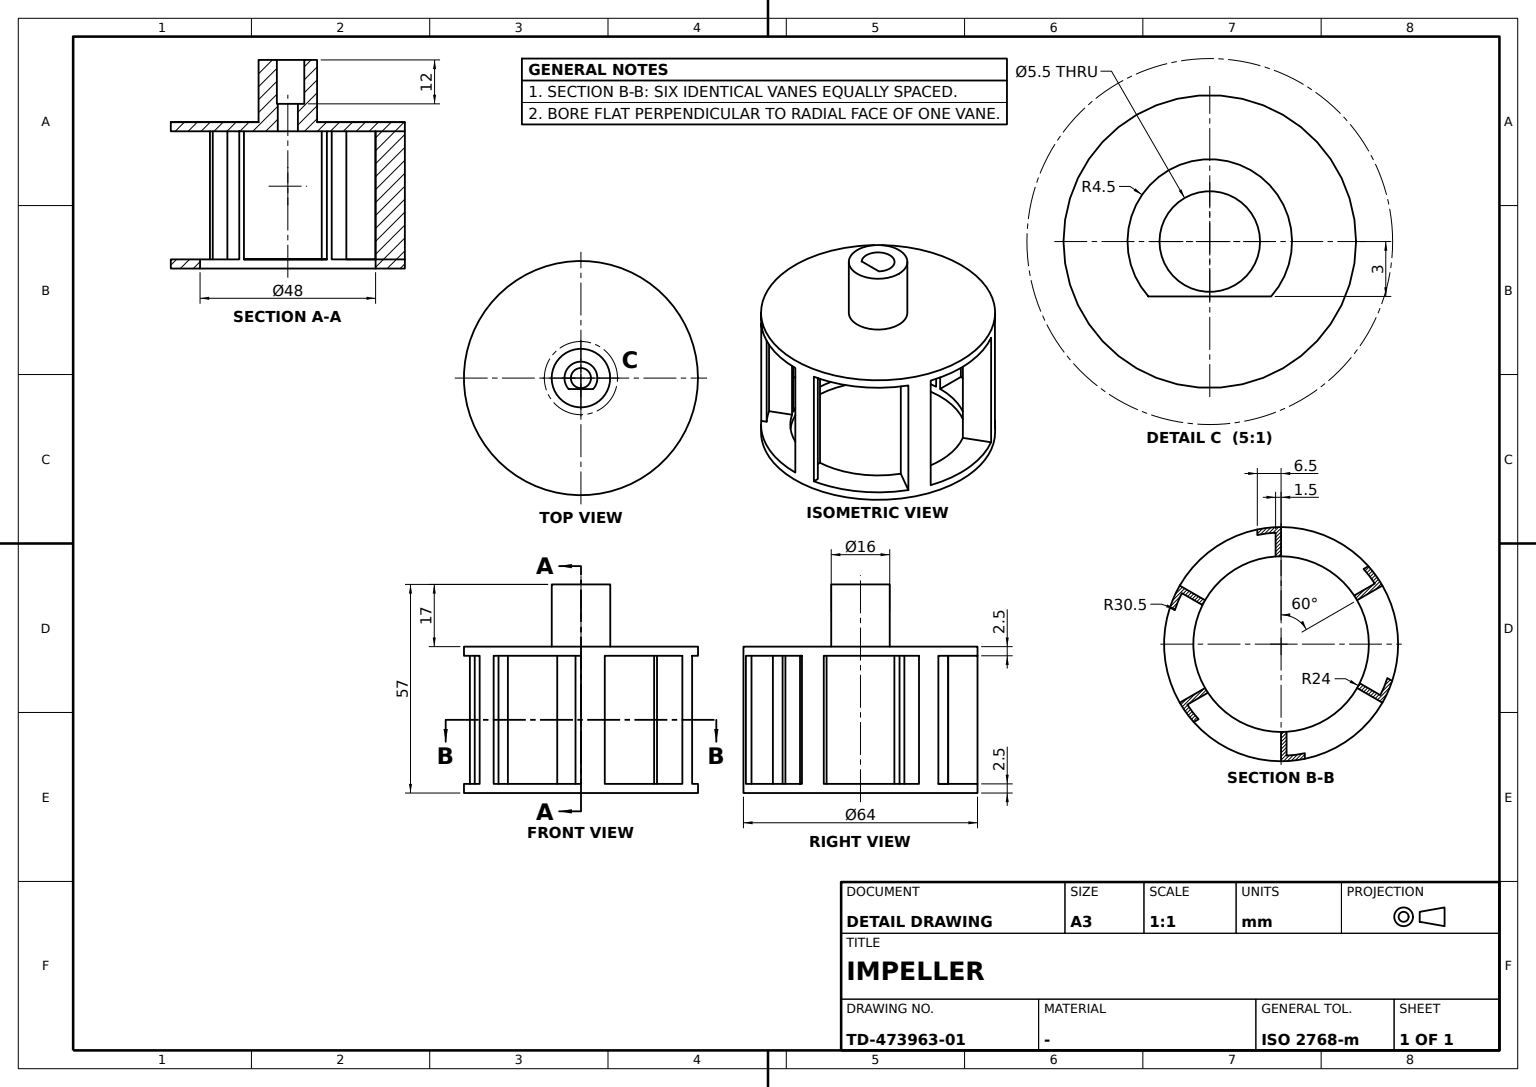
ISO-10303-21;
HEADER;
FILE_DESCRIPTION((''),'2;1');
FILE_NAME('','',(''),(''),'','','');
FILE_SCHEMA(('AUTOMOTIVE_DESIGN'));
ENDSEC;
DATA;
#1=APPLICATION_CONTEXT('');
#2=PRODUCT_CONTEXT('',#1,'mechanical');
#3=PRODUCT('','','',(#2));
#4=PRODUCT_DEFINITION_FORMATION('','',#3);
#5=PRODUCT_DEFINITION_CONTEXT('',#1,'design');
#6=PRODUCT_DEFINITION('','',#4,#5);
#7=PRODUCT_DEFINITION_SHAPE('','',#6);
#8=(LENGTH_UNIT()NAMED_UNIT(*)SI_UNIT(.MILLI.,.METRE.));
#9=(NAMED_UNIT(*)PLANE_ANGLE_UNIT()SI_UNIT($,.RADIAN.));
#10=(NAMED_UNIT(*)SI_UNIT($,.STERADIAN.)SOLID_ANGLE_UNIT());
#11=UNCERTAINTY_MEASURE_WITH_UNIT(LENGTH_MEASURE(0.005),#8,'distance_accuracy_value','');
#12=(GEOMETRIC_REPRESENTATION_CONTEXT(3)GLOBAL_UNCERTAINTY_ASSIGNED_CONTEXT((#11))GLOBAL_UNIT_ASSIGNED_CONTEXT((#8,#9,#10))REPRESENTATION_CONTEXT('',''));
#13=CARTESIAN_POINT('',(20.78461,12.,2.5));
#14=VERTEX_POINT('',#13);
#15=CARTESIAN_POINT('',(20.78461,12.,37.5));
#16=VERTEX_POINT('',#15);
#17=DIRECTION('',(0.,0.,1.));
#18=VECTOR('',#17,1000.);
#19=LINE('',#13,#18);
#20=EDGE_CURVE('',#14,#16,#19,.T.);
#21=ORIENTED_EDGE('',*,*,#20,.T.);
#22=CARTESIAN_POINT('',(27.712813,16.,37.5));
#23=VERTEX_POINT('',#22);
#24=CARTESIAN_POINT('',(0.,0.,37.5));
#25=DIRECTION('',(0.866025404,0.5,0.));
#26=VECTOR('',#25,1000.);
#27=LINE('',#24,#26);
#28=EDGE_CURVE('',#16,#23,#27,.T.);
#29=ORIENTED_EDGE('',*,*,#28,.T.);
#30=CARTESIAN_POINT('',(27.712813,16.,2.5));
#31=VERTEX_POINT('',#30);
#32=LINE('',#30,#18);
#33=EDGE_CURVE('',#31,#23,#32,.T.);
#34=ORIENTED_EDGE('',*,*,#33,.F.);
#35=CARTESIAN_POINT('',(0.,0.,2.5));
#36=LINE('',#35,#26);
#37=EDGE_CURVE('',#14,#31,#36,.T.);
#38=ORIENTED_EDGE('',*,*,#37,.F.);
#39=EDGE_LOOP('',(#21,#29,#34,#38));
#40=FACE_BOUND('',#39,.T.);
#41=DIRECTION('',(0.5,-0.866025404,0.));
#42=AXIS2_PLACEMENT_3D('',#13,#41,#25);
#43=PLANE('',#42);
#44=ADVANCED_FACE('',(#40),#43,.F.);
#45=CARTESIAN_POINT('',(29.056976,9.270499,2.5));
#46=VERTEX_POINT('',#45);
#47=CARTESIAN_POINT('',(29.056976,9.270499,37.5));
#48=VERTEX_POINT('',#47);
#49=LINE('',#45,#18);
#50=EDGE_CURVE('',#46,#48,#49,.T.);
#51=ORIENTED_EDGE('',*,*,#50,.T.);
#52=CARTESIAN_POINT('',(27.131812,13.932508,37.5));
#53=VERTEX_POINT('',#52);
#54=DIRECTION('',(1.,0.,0.));
#55=AXIS2_PLACEMENT_3D('',#24,#17,#54);
#56=CIRCLE('',#55,30.5);
#57=EDGE_CURVE('',#48,#53,#56,.T.);
#58=ORIENTED_EDGE('',*,*,#57,.T.);
#59=CARTESIAN_POINT('',(27.131812,13.932508,2.5));
#60=VERTEX_POINT('',#59);
#61=LINE('',#59,#18);
#62=EDGE_CURVE('',#60,#53,#61,.T.);
#63=ORIENTED_EDGE('',*,*,#62,.F.);
#64=AXIS2_PLACEMENT_3D('',#35,#17,#54);
#65=CIRCLE('',#64,30.5);
#66=EDGE_CURVE('',#46,#60,#65,.T.);
#67=ORIENTED_EDGE('',*,*,#66,.F.);
#68=EDGE_LOOP('',(#51,#58,#63,#67));
#69=FACE_BOUND('',#68,.T.);
#70=CARTESIAN_POINT('',(0.,0.,20.5));
#71=DIRECTION('',(-0.866025404,0.5,0.));
#72=AXIS2_PLACEMENT_3D('',#70,#17,#71);
#73=CYLINDRICAL_SURFACE('',#72,30.5);
#74=ADVANCED_FACE('',(#69),#73,.F.);
#75=CARTESIAN_POINT('',(21.493975,10.677501,2.5));
#76=VERTEX_POINT('',#75);
#77=CARTESIAN_POINT('',(0.75,-1.299038,2.5));
#78=DIRECTION('',(-0.866025404,-0.5,0.));
#79=VECTOR('',#78,1000.);
#80=LINE('',#77,#79);
#81=EDGE_CURVE('',#60,#76,#80,.T.);
#82=ORIENTED_EDGE('',*,*,#81,.F.);
#83=ORIENTED_EDGE('',*,*,#62,.T.);
#84=CARTESIAN_POINT('',(21.493975,10.677501,37.5));
#85=VERTEX_POINT('',#84);
#86=CARTESIAN_POINT('',(0.75,-1.299038,37.5));
#87=LINE('',#86,#79);
#88=EDGE_CURVE('',#53,#85,#87,.T.);
#89=ORIENTED_EDGE('',*,*,#88,.T.);
#90=LINE('',#75,#18);
#91=EDGE_CURVE('',#76,#85,#90,.T.);
#92=ORIENTED_EDGE('',*,*,#91,.F.);
#93=EDGE_LOOP('',(#82,#83,#89,#92));
#94=FACE_BOUND('',#93,.T.);
#95=DIRECTION('',(-0.5,0.866025404,0.));
#96=AXIS2_PLACEMENT_3D('',#59,#95,#78);
#97=PLANE('',#96);
#98=ADVANCED_FACE('',(#94),#97,.F.);
#99=CARTESIAN_POINT('',(8.,0.,0.));
#100=VERTEX_POINT('',#99);
#101=CARTESIAN_POINT('',(0.,0.,0.));
#102=AXIS2_PLACEMENT_3D('',#101,#17,#54);
#103=CIRCLE('',#102,8.);
#104=EDGE_CURVE('',#100,#100,#103,.F.);
#105=ORIENTED_EDGE('',*,*,#104,.F.);
#106=EDGE_LOOP('',(#105));
#107=FACE_BOUND('',#106,.T.);
#108=CARTESIAN_POINT('',(32.,0.,0.));
#109=VERTEX_POINT('',#108);
#110=CIRCLE('',#102,32.);
#111=EDGE_CURVE('',#109,#109,#110,.T.);
#112=ORIENTED_EDGE('',*,*,#111,.F.);
#113=EDGE_LOOP('',(#112));
#114=FACE_BOUND('',#113,.T.);
#115=DIRECTION('',(0.,1.,0.));
#116=AXIS2_PLACEMENT_3D('',#101,#17,#115);
#117=PLANE('',#116);
#118=ADVANCED_FACE('',(#107,#114),#117,.F.);
#119=CARTESIAN_POINT('',(-1.5,-30.463092,37.5));
#120=VERTEX_POINT('',#119);
#121=CARTESIAN_POINT('',(-1.5,-23.953079,37.5));
#122=VERTEX_POINT('',#121);
#123=CARTESIAN_POINT('',(-1.5,0.,37.5));
#124=VECTOR('',#115,1000.);
#125=LINE('',#123,#124);
#126=EDGE_CURVE('',#120,#122,#125,.T.);
#127=ORIENTED_EDGE('',*,*,#126,.T.);
#128=CARTESIAN_POINT('',(-1.5,-23.953079,2.5));
#129=VERTEX_POINT('',#128);
#130=LINE('',#128,#18);
#131=EDGE_CURVE('',#129,#122,#130,.T.);
#132=ORIENTED_EDGE('',*,*,#131,.F.);
#133=CARTESIAN_POINT('',(-1.5,-30.463092,2.5));
#134=VERTEX_POINT('',#133);
#135=CARTESIAN_POINT('',(-1.5,0.,2.5));
#136=LINE('',#135,#124);
#137=EDGE_CURVE('',#134,#129,#136,.T.);
#138=ORIENTED_EDGE('',*,*,#137,.F.);
#139=LINE('',#133,#18);
#140=EDGE_CURVE('',#134,#120,#139,.T.);
#141=ORIENTED_EDGE('',*,*,#140,.T.);
#142=EDGE_LOOP('',(#127,#132,#138,#141));
#143=FACE_BOUND('',#142,.T.);
#144=AXIS2_PLACEMENT_3D('',#133,#54,#115);
#145=PLANE('',#144);
#146=ADVANCED_FACE('',(#143),#145,.F.);
#147=CARTESIAN_POINT('',(32.,0.,40.));
#148=VERTEX_POINT('',#147);
#149=CARTESIAN_POINT('',(0.,0.,40.));
#150=AXIS2_PLACEMENT_3D('',#149,#17,#54);
#151=CIRCLE('',#150,32.);
#152=EDGE_CURVE('',#148,#148,#151,.T.);
#153=ORIENTED_EDGE('',*,*,#152,.T.);
#154=EDGE_LOOP('',(#153));
#155=FACE_BOUND('',#154,.T.);
#156=CARTESIAN_POINT('',(24.,0.,40.));
#157=VERTEX_POINT('',#156);
#158=CIRCLE('',#150,24.);
#159=EDGE_CURVE('',#157,#157,#158,.T.);
#160=ORIENTED_EDGE('',*,*,#159,.F.);
#161=EDGE_LOOP('',(#160));
#162=FACE_BOUND('',#161,.T.);
#163=AXIS2_PLACEMENT_3D('',#149,#17,#115);
#164=PLANE('',#163);
#165=ADVANCED_FACE('',(#155,#162),#164,.T.);
#166=CARTESIAN_POINT('',(25.631812,-16.530584,2.5));
#167=VERTEX_POINT('',#166);
#168=CARTESIAN_POINT('',(25.631812,-16.530584,37.5));
#169=VERTEX_POINT('',#168);
#170=LINE('',#166,#18);
#171=EDGE_CURVE('',#167,#169,#170,.T.);
#172=ORIENTED_EDGE('',*,*,#171,.T.);
#173=CARTESIAN_POINT('',(19.993975,-13.275578,37.5));
#174=VERTEX_POINT('',#173);
#175=CARTESIAN_POINT('',(-0.75,-1.299038,37.5));
#176=VECTOR('',#71,1000.);
#177=LINE('',#175,#176);
#178=EDGE_CURVE('',#169,#174,#177,.T.);
#179=ORIENTED_EDGE('',*,*,#178,.T.);
#180=CARTESIAN_POINT('',(19.993975,-13.275578,2.5));
#181=VERTEX_POINT('',#180);
#182=LINE('',#180,#18);
#183=EDGE_CURVE('',#181,#174,#182,.T.);
#184=ORIENTED_EDGE('',*,*,#183,.F.);
#185=CARTESIAN_POINT('',(-0.75,-1.299038,2.5));
#186=LINE('',#185,#176);
#187=EDGE_CURVE('',#167,#181,#186,.T.);
#188=ORIENTED_EDGE('',*,*,#187,.F.);
#189=EDGE_LOOP('',(#172,#179,#184,#188));
#190=FACE_BOUND('',#189,.T.);
#191=DIRECTION('',(0.5,0.866025404,0.));
#192=AXIS2_PLACEMENT_3D('',#166,#191,#71);
#193=PLANE('',#192);
#194=ADVANCED_FACE('',(#190),#193,.F.);
#195=CARTESIAN_POINT('',(-22.556976,20.52883,37.5));
#196=VERTEX_POINT('',#195);
#197=CARTESIAN_POINT('',(-23.885079,21.29561,37.5));
#198=VERTEX_POINT('',#197);
#199=CARTESIAN_POINT('',(3.25,5.629165,37.5));
#200=LINE('',#199,#176);
#201=EDGE_CURVE('',#196,#198,#200,.T.);
#202=ORIENTED_EDGE('',*,*,#201,.T.);
#203=CARTESIAN_POINT('',(0.,32.,37.5));
#204=VERTEX_POINT('',#203);
#205=CIRCLE('',#55,32.);
#206=EDGE_CURVE('',#204,#198,#205,.T.);
#207=ORIENTED_EDGE('',*,*,#206,.F.);
#208=CARTESIAN_POINT('',(0.,24.,37.5));
#209=VERTEX_POINT('',#208);
#210=DIRECTION('',(0.,-1.,0.));
#211=VECTOR('',#210,1000.);
#212=LINE('',#208,#211);
#213=EDGE_CURVE('',#204,#209,#212,.T.);
#214=ORIENTED_EDGE('',*,*,#213,.T.);
#215=CARTESIAN_POINT('',(-19.993975,13.275578,37.5));
#216=VERTEX_POINT('',#215);
#217=CIRCLE('',#55,24.);
#218=EDGE_CURVE('',#209,#216,#217,.T.);
#219=ORIENTED_EDGE('',*,*,#218,.T.);
#220=CARTESIAN_POINT('',(-25.631812,16.530584,37.5));
#221=VERTEX_POINT('',#220);
#222=CARTESIAN_POINT('',(0.75,1.299038,37.5));
#223=DIRECTION('',(0.866025404,-0.5,0.));
#224=VECTOR('',#223,1000.);
#225=LINE('',#222,#224);
#226=EDGE_CURVE('',#221,#216,#225,.T.);
#227=ORIENTED_EDGE('',*,*,#226,.F.);
#228=EDGE_CURVE('',#196,#221,#56,.T.);
#229=ORIENTED_EDGE('',*,*,#228,.F.);
#230=EDGE_LOOP('',(#202,#207,#214,#219,#227,#229));
#231=FACE_BOUND('',#230,.T.);
#232=AXIS2_PLACEMENT_3D('',#24,#17,#115);
#233=PLANE('',#232);
#234=ADVANCED_FACE('',(#231),#233,.F.);
#235=CARTESIAN_POINT('',(-3.354102,3.,-17.));
#236=VERTEX_POINT('',#235);
#237=CARTESIAN_POINT('',(3.354102,3.,-17.));
#238=VERTEX_POINT('',#237);
#239=VECTOR('',#54,1000.);
#240=LINE('',#235,#239);
#241=EDGE_CURVE('',#236,#238,#240,.T.);
#242=ORIENTED_EDGE('',*,*,#241,.F.);
#243=CARTESIAN_POINT('',(0.,0.,-17.));
#244=DIRECTION('',(0.,0.,-1.));
#245=DIRECTION('',(-1.,0.,0.));
#246=AXIS2_PLACEMENT_3D('',#243,#244,#245);
#247=CIRCLE('',#246,4.5);
#248=EDGE_CURVE('',#238,#236,#247,.T.);
#249=ORIENTED_EDGE('',*,*,#248,.F.);
#250=EDGE_LOOP('',(#242,#249));
#251=FACE_BOUND('',#250,.T.);
#252=CARTESIAN_POINT('',(-8.,0.,-17.));
#253=VERTEX_POINT('',#252);
#254=CIRCLE('',#246,8.);
#255=EDGE_CURVE('',#253,#253,#254,.T.);
#256=ORIENTED_EDGE('',*,*,#255,.T.);
#257=EDGE_LOOP('',(#256));
#258=FACE_BOUND('',#257,.T.);
#259=AXIS2_PLACEMENT_3D('',#243,#244,#54);
#260=PLANE('',#259);
#261=ADVANCED_FACE('',(#251,#258),#260,.T.);
#262=CARTESIAN_POINT('',(6.5,29.799329,37.5));
#263=VERTEX_POINT('',#262);
#264=CARTESIAN_POINT('',(6.5,31.33289,37.5));
#265=VERTEX_POINT('',#264);
#266=CARTESIAN_POINT('',(6.5,0.,37.5));
#267=LINE('',#266,#124);
#268=EDGE_CURVE('',#263,#265,#267,.T.);
#269=ORIENTED_EDGE('',*,*,#268,.F.);
#270=CARTESIAN_POINT('',(6.5,29.799329,2.5));
#271=VERTEX_POINT('',#270);
#272=LINE('',#270,#18);
#273=EDGE_CURVE('',#271,#263,#272,.T.);
#274=ORIENTED_EDGE('',*,*,#273,.F.);
#275=CARTESIAN_POINT('',(6.5,31.33289,2.5));
#276=VERTEX_POINT('',#275);
#277=CARTESIAN_POINT('',(6.5,0.,2.5));
#278=LINE('',#277,#124);
#279=EDGE_CURVE('',#271,#276,#278,.T.);
#280=ORIENTED_EDGE('',*,*,#279,.T.);
#281=LINE('',#275,#18);
#282=EDGE_CURVE('',#276,#265,#281,.T.);
#283=ORIENTED_EDGE('',*,*,#282,.T.);
#284=EDGE_LOOP('',(#269,#274,#280,#283));
#285=FACE_BOUND('',#284,.T.);
#286=AXIS2_PLACEMENT_3D('',#270,#54,#115);
#287=PLANE('',#286);
#288=ADVANCED_FACE('',(#285),#287,.T.);
#289=CARTESIAN_POINT('',(0.,-32.,2.5));
#290=VERTEX_POINT('',#289);
#291=CARTESIAN_POINT('',(0.,-32.,37.5));
#292=VERTEX_POINT('',#291);
#293=LINE('',#289,#18);
#294=EDGE_CURVE('',#290,#292,#293,.T.);
#295=ORIENTED_EDGE('',*,*,#294,.F.);
#296=CARTESIAN_POINT('',(0.,-24.,2.5));
#297=VERTEX_POINT('',#296);
#298=LINE('',#35,#124);
#299=EDGE_CURVE('',#290,#297,#298,.T.);
#300=ORIENTED_EDGE('',*,*,#299,.T.);
#301=CARTESIAN_POINT('',(0.,-24.,37.5));
#302=VERTEX_POINT('',#301);
#303=LINE('',#296,#18);
#304=EDGE_CURVE('',#297,#302,#303,.T.);
#305=ORIENTED_EDGE('',*,*,#304,.T.);
#306=LINE('',#24,#124);
#307=EDGE_CURVE('',#292,#302,#306,.T.);
#308=ORIENTED_EDGE('',*,*,#307,.F.);
#309=EDGE_LOOP('',(#295,#300,#305,#308));
#310=FACE_BOUND('',#309,.T.);
#311=CARTESIAN_POINT('',(0.,24.,2.5));
#312=AXIS2_PLACEMENT_3D('',#311,#54,#115);
#313=PLANE('',#312);
#314=ADVANCED_FACE('',(#310),#313,.T.);
#315=ORIENTED_EDGE('',*,*,#57,.F.);
#316=CARTESIAN_POINT('',(30.385079,10.03728,37.5));
#317=VERTEX_POINT('',#316);
#318=CARTESIAN_POINT('',(3.25,-5.629165,37.5));
#319=LINE('',#318,#26);
#320=EDGE_CURVE('',#48,#317,#319,.T.);
#321=ORIENTED_EDGE('',*,*,#320,.T.);
#322=CARTESIAN_POINT('',(27.712813,-16.,37.5));
#323=VERTEX_POINT('',#322);
#324=EDGE_CURVE('',#323,#317,#205,.T.);
#325=ORIENTED_EDGE('',*,*,#324,.F.);
#326=CARTESIAN_POINT('',(20.78461,-12.,37.5));
#327=VERTEX_POINT('',#326);
#328=LINE('',#24,#176);
#329=EDGE_CURVE('',#327,#323,#328,.F.);
#330=ORIENTED_EDGE('',*,*,#329,.F.);
#331=EDGE_CURVE('',#327,#85,#217,.T.);
#332=ORIENTED_EDGE('',*,*,#331,.T.);
#333=ORIENTED_EDGE('',*,*,#88,.F.);
#334=EDGE_LOOP('',(#315,#321,#325,#330,#332,#333));
#335=FACE_BOUND('',#334,.T.);
#336=ADVANCED_FACE('',(#335),#233,.F.);
#337=CARTESIAN_POINT('',(-6.5,-29.799329,37.5));
#338=VERTEX_POINT('',#337);
#339=CARTESIAN_POINT('',(-6.5,-31.33289,37.5));
#340=VERTEX_POINT('',#339);
#341=CARTESIAN_POINT('',(-6.5,0.,37.5));
#342=LINE('',#341,#211);
#343=EDGE_CURVE('',#338,#340,#342,.T.);
#344=ORIENTED_EDGE('',*,*,#343,.F.);
#345=CARTESIAN_POINT('',(-6.5,-29.799329,2.5));
#346=VERTEX_POINT('',#345);
#347=LINE('',#345,#18);
#348=EDGE_CURVE('',#346,#338,#347,.T.);
#349=ORIENTED_EDGE('',*,*,#348,.F.);
#350=CARTESIAN_POINT('',(-6.5,-31.33289,2.5));
#351=VERTEX_POINT('',#350);
#352=CARTESIAN_POINT('',(-6.5,0.,2.5));
#353=LINE('',#352,#211);
#354=EDGE_CURVE('',#346,#351,#353,.T.);
#355=ORIENTED_EDGE('',*,*,#354,.T.);
#356=LINE('',#350,#18);
#357=EDGE_CURVE('',#351,#340,#356,.T.);
#358=ORIENTED_EDGE('',*,*,#357,.T.);
#359=EDGE_LOOP('',(#344,#349,#355,#358));
#360=FACE_BOUND('',#359,.T.);
#361=AXIS2_PLACEMENT_3D('',#345,#245,#210);
#362=PLANE('',#361);
#363=ADVANCED_FACE('',(#360),#362,.T.);
#364=CARTESIAN_POINT('',(-2.75,0.,-5.));
#365=VERTEX_POINT('',#364);
#366=CARTESIAN_POINT('',(0.,0.,-5.));
#367=AXIS2_PLACEMENT_3D('',#366,#244,#245);
#368=CIRCLE('',#367,2.75);
#369=EDGE_CURVE('',#365,#365,#368,.T.);
#370=ORIENTED_EDGE('',*,*,#369,.T.);
#371=EDGE_LOOP('',(#370));
#372=FACE_BOUND('',#371,.T.);
#373=CARTESIAN_POINT('',(2.75,0.,2.5));
#374=VERTEX_POINT('',#373);
#375=CIRCLE('',#64,2.75);
#376=EDGE_CURVE('',#374,#374,#375,.T.);
#377=ORIENTED_EDGE('',*,*,#376,.T.);
#378=EDGE_LOOP('',(#377));
#379=FACE_BOUND('',#378,.T.);
#380=CARTESIAN_POINT('',(0.,0.,18.16));
#381=AXIS2_PLACEMENT_3D('',#380,#244,#54);
#382=CYLINDRICAL_SURFACE('',#381,2.75);
#383=ADVANCED_FACE('',(#372,#379),#382,.F.);
#384=ORIENTED_EDGE('',*,*,#320,.F.);
#385=ORIENTED_EDGE('',*,*,#50,.F.);
#386=CARTESIAN_POINT('',(30.385079,10.03728,2.5));
#387=VERTEX_POINT('',#386);
#388=CARTESIAN_POINT('',(3.25,-5.629165,2.5));
#389=LINE('',#388,#26);
#390=EDGE_CURVE('',#46,#387,#389,.T.);
#391=ORIENTED_EDGE('',*,*,#390,.T.);
#392=LINE('',#386,#18);
#393=EDGE_CURVE('',#387,#317,#392,.T.);
#394=ORIENTED_EDGE('',*,*,#393,.T.);
#395=EDGE_LOOP('',(#384,#385,#391,#394));
#396=FACE_BOUND('',#395,.T.);
#397=AXIS2_PLACEMENT_3D('',#45,#41,#25);
#398=PLANE('',#397);
#399=ADVANCED_FACE('',(#396),#398,.T.);
#400=CARTESIAN_POINT('',(-27.712813,16.,2.5));
#401=VERTEX_POINT('',#400);
#402=CARTESIAN_POINT('',(-27.712813,16.,37.5));
#403=VERTEX_POINT('',#402);
#404=LINE('',#400,#18);
#405=EDGE_CURVE('',#401,#403,#404,.T.);
#406=ORIENTED_EDGE('',*,*,#405,.F.);
#407=CARTESIAN_POINT('',(-20.78461,12.,2.5));
#408=VERTEX_POINT('',#407);
#409=LINE('',#35,#176);
#410=EDGE_CURVE('',#408,#401,#409,.T.);
#411=ORIENTED_EDGE('',*,*,#410,.F.);
#412=CARTESIAN_POINT('',(-20.78461,12.,37.5));
#413=VERTEX_POINT('',#412);
#414=LINE('',#407,#18);
#415=EDGE_CURVE('',#408,#413,#414,.T.);
#416=ORIENTED_EDGE('',*,*,#415,.T.);
#417=EDGE_CURVE('',#413,#403,#328,.T.);
#418=ORIENTED_EDGE('',*,*,#417,.T.);
#419=EDGE_LOOP('',(#406,#411,#416,#418));
#420=FACE_BOUND('',#419,.T.);
#421=AXIS2_PLACEMENT_3D('',#407,#191,#71);
#422=PLANE('',#421);
#423=ADVANCED_FACE('',(#420),#422,.F.);
#424=ORIENTED_EDGE('',*,*,#268,.T.);
#425=EDGE_CURVE('',#23,#265,#205,.T.);
#426=ORIENTED_EDGE('',*,*,#425,.F.);
#427=ORIENTED_EDGE('',*,*,#28,.F.);
#428=CARTESIAN_POINT('',(1.5,23.953079,37.5));
#429=VERTEX_POINT('',#428);
#430=EDGE_CURVE('',#16,#429,#217,.T.);
#431=ORIENTED_EDGE('',*,*,#430,.T.);
#432=CARTESIAN_POINT('',(1.5,30.463092,37.5));
#433=VERTEX_POINT('',#432);
#434=CARTESIAN_POINT('',(1.5,0.,37.5));
#435=LINE('',#434,#211);
#436=EDGE_CURVE('',#433,#429,#435,.T.);
#437=ORIENTED_EDGE('',*,*,#436,.F.);
#438=EDGE_CURVE('',#263,#433,#56,.T.);
#439=ORIENTED_EDGE('',*,*,#438,.F.);
#440=EDGE_LOOP('',(#424,#426,#427,#431,#437,#439));
#441=FACE_BOUND('',#440,.T.);
#442=ADVANCED_FACE('',(#441),#233,.F.);
#443=CARTESIAN_POINT('',(-20.78461,-12.,2.5));
#444=VERTEX_POINT('',#443);
#445=CARTESIAN_POINT('',(-27.712813,-16.,2.5));
#446=VERTEX_POINT('',#445);
#447=EDGE_CURVE('',#444,#446,#36,.F.);
#448=ORIENTED_EDGE('',*,*,#447,.F.);
#449=CARTESIAN_POINT('',(-20.78461,-12.,37.5));
#450=VERTEX_POINT('',#449);
#451=LINE('',#443,#18);
#452=EDGE_CURVE('',#444,#450,#451,.T.);
#453=ORIENTED_EDGE('',*,*,#452,.T.);
#454=CARTESIAN_POINT('',(-27.712813,-16.,37.5));
#455=VERTEX_POINT('',#454);
#456=EDGE_CURVE('',#450,#455,#27,.F.);
#457=ORIENTED_EDGE('',*,*,#456,.T.);
#458=LINE('',#445,#18);
#459=EDGE_CURVE('',#446,#455,#458,.T.);
#460=ORIENTED_EDGE('',*,*,#459,.F.);
#461=EDGE_LOOP('',(#448,#453,#457,#460));
#462=FACE_BOUND('',#461,.T.);
#463=ADVANCED_FACE('',(#462),#43,.T.);
#464=CARTESIAN_POINT('',(-27.131812,-13.932508,37.5));
#465=VERTEX_POINT('',#464);
#466=CARTESIAN_POINT('',(-21.493975,-10.677501,37.5));
#467=VERTEX_POINT('',#466);
#468=CARTESIAN_POINT('',(-0.75,1.299038,37.5));
#469=LINE('',#468,#26);
#470=EDGE_CURVE('',#465,#467,#469,.T.);
#471=ORIENTED_EDGE('',*,*,#470,.T.);
#472=CARTESIAN_POINT('',(-21.493975,-10.677501,2.5));
#473=VERTEX_POINT('',#472);
#474=LINE('',#472,#18);
#475=EDGE_CURVE('',#473,#467,#474,.T.);
#476=ORIENTED_EDGE('',*,*,#475,.F.);
#477=CARTESIAN_POINT('',(-27.131812,-13.932508,2.5));
#478=VERTEX_POINT('',#477);
#479=CARTESIAN_POINT('',(-0.75,1.299038,2.5));
#480=LINE('',#479,#26);
#481=EDGE_CURVE('',#478,#473,#480,.T.);
#482=ORIENTED_EDGE('',*,*,#481,.F.);
#483=LINE('',#477,#18);
#484=EDGE_CURVE('',#478,#465,#483,.T.);
#485=ORIENTED_EDGE('',*,*,#484,.T.);
#486=EDGE_LOOP('',(#471,#476,#482,#485));
#487=FACE_BOUND('',#486,.T.);
#488=AXIS2_PLACEMENT_3D('',#477,#41,#25);
#489=PLANE('',#488);
#490=ADVANCED_FACE('',(#487),#489,.F.);
#491=ORIENTED_EDGE('',*,*,#329,.T.);
#492=CARTESIAN_POINT('',(27.712813,-16.,2.5));
#493=VERTEX_POINT('',#492);
#494=LINE('',#492,#18);
#495=EDGE_CURVE('',#493,#323,#494,.T.);
#496=ORIENTED_EDGE('',*,*,#495,.F.);
#497=CARTESIAN_POINT('',(20.78461,-12.,2.5));
#498=VERTEX_POINT('',#497);
#499=EDGE_CURVE('',#498,#493,#409,.F.);
#500=ORIENTED_EDGE('',*,*,#499,.F.);
#501=LINE('',#497,#18);
#502=EDGE_CURVE('',#498,#327,#501,.T.);
#503=ORIENTED_EDGE('',*,*,#502,.T.);
#504=EDGE_LOOP('',(#491,#496,#500,#503));
#505=FACE_BOUND('',#504,.T.);
#506=ADVANCED_FACE('',(#505),#422,.T.);
#507=ORIENTED_EDGE('',*,*,#171,.F.);
#508=CARTESIAN_POINT('',(22.556976,-20.52883,2.5));
#509=VERTEX_POINT('',#508);
#510=EDGE_CURVE('',#509,#167,#65,.T.);
#511=ORIENTED_EDGE('',*,*,#510,.F.);
#512=CARTESIAN_POINT('',(22.556976,-20.52883,37.5));
#513=VERTEX_POINT('',#512);
#514=LINE('',#508,#18);
#515=EDGE_CURVE('',#509,#513,#514,.T.);
#516=ORIENTED_EDGE('',*,*,#515,.T.);
#517=EDGE_CURVE('',#513,#169,#56,.T.);
#518=ORIENTED_EDGE('',*,*,#517,.T.);
#519=EDGE_LOOP('',(#507,#511,#516,#518));
#520=FACE_BOUND('',#519,.T.);
#521=ADVANCED_FACE('',(#520),#73,.F.);
#522=CARTESIAN_POINT('',(-25.631812,16.530584,2.5));
#523=VERTEX_POINT('',#522);
#524=CARTESIAN_POINT('',(-19.993975,13.275578,2.5));
#525=VERTEX_POINT('',#524);
#526=CARTESIAN_POINT('',(0.75,1.299038,2.5));
#527=LINE('',#526,#224);
#528=EDGE_CURVE('',#523,#525,#527,.T.);
#529=ORIENTED_EDGE('',*,*,#528,.F.);
#530=LINE('',#522,#18);
#531=EDGE_CURVE('',#523,#221,#530,.T.);
#532=ORIENTED_EDGE('',*,*,#531,.T.);
#533=ORIENTED_EDGE('',*,*,#226,.T.);
#534=LINE('',#524,#18);
#535=EDGE_CURVE('',#525,#216,#534,.T.);
#536=ORIENTED_EDGE('',*,*,#535,.F.);
#537=EDGE_LOOP('',(#529,#532,#533,#536));
#538=FACE_BOUND('',#537,.T.);
#539=DIRECTION('',(-0.5,-0.866025404,0.));
#540=AXIS2_PLACEMENT_3D('',#522,#539,#223);
#541=PLANE('',#540);
#542=ADVANCED_FACE('',(#538),#541,.F.);
#543=CARTESIAN_POINT('',(-29.056976,-9.270499,37.5));
#544=VERTEX_POINT('',#543);
#545=CARTESIAN_POINT('',(-30.385079,-10.03728,37.5));
#546=VERTEX_POINT('',#545);
#547=CARTESIAN_POINT('',(-3.25,5.629165,37.5));
#548=LINE('',#547,#79);
#549=EDGE_CURVE('',#544,#546,#548,.T.);
#550=ORIENTED_EDGE('',*,*,#549,.F.);
#551=CARTESIAN_POINT('',(-29.056976,-9.270499,2.5));
#552=VERTEX_POINT('',#551);
#553=LINE('',#551,#18);
#554=EDGE_CURVE('',#552,#544,#553,.T.);
#555=ORIENTED_EDGE('',*,*,#554,.F.);
#556=CARTESIAN_POINT('',(-30.385079,-10.03728,2.5));
#557=VERTEX_POINT('',#556);
#558=CARTESIAN_POINT('',(-3.25,5.629165,2.5));
#559=LINE('',#558,#79);
#560=EDGE_CURVE('',#552,#557,#559,.T.);
#561=ORIENTED_EDGE('',*,*,#560,.T.);
#562=LINE('',#556,#18);
#563=EDGE_CURVE('',#557,#546,#562,.T.);
#564=ORIENTED_EDGE('',*,*,#563,.T.);
#565=EDGE_LOOP('',(#550,#555,#561,#564));
#566=FACE_BOUND('',#565,.T.);
#567=AXIS2_PLACEMENT_3D('',#551,#95,#78);
#568=PLANE('',#567);
#569=ADVANCED_FACE('',(#566),#568,.T.);
#570=CARTESIAN_POINT('',(-3.354102,3.,-5.));
#571=VERTEX_POINT('',#570);
#572=CARTESIAN_POINT('',(3.354102,3.,-5.));
#573=VERTEX_POINT('',#572);
#574=LINE('',#570,#239);
#575=EDGE_CURVE('',#571,#573,#574,.T.);
#576=ORIENTED_EDGE('',*,*,#575,.F.);
#577=VECTOR('',#244,1000.);
#578=LINE('',#235,#577);
#579=EDGE_CURVE('',#571,#236,#578,.T.);
#580=ORIENTED_EDGE('',*,*,#579,.T.);
#581=ORIENTED_EDGE('',*,*,#241,.T.);
#582=LINE('',#237,#577);
#583=EDGE_CURVE('',#238,#573,#582,.F.);
#584=ORIENTED_EDGE('',*,*,#583,.T.);
#585=EDGE_LOOP('',(#576,#580,#581,#584));
#586=FACE_BOUND('',#585,.T.);
#587=AXIS2_PLACEMENT_3D('',#235,#210,#54);
#588=PLANE('',#587);
#589=ADVANCED_FACE('',(#586),#588,.T.);
#590=ORIENTED_EDGE('',*,*,#201,.F.);
#591=CARTESIAN_POINT('',(-22.556976,20.52883,2.5));
#592=VERTEX_POINT('',#591);
#593=LINE('',#591,#18);
#594=EDGE_CURVE('',#592,#196,#593,.T.);
#595=ORIENTED_EDGE('',*,*,#594,.F.);
#596=CARTESIAN_POINT('',(-23.885079,21.29561,2.5));
#597=VERTEX_POINT('',#596);
#598=CARTESIAN_POINT('',(3.25,5.629165,2.5));
#599=LINE('',#598,#176);
#600=EDGE_CURVE('',#592,#597,#599,.T.);
#601=ORIENTED_EDGE('',*,*,#600,.T.);
#602=LINE('',#596,#18);
#603=EDGE_CURVE('',#597,#198,#602,.T.);
#604=ORIENTED_EDGE('',*,*,#603,.T.);
#605=EDGE_LOOP('',(#590,#595,#601,#604));
#606=FACE_BOUND('',#605,.T.);
#607=AXIS2_PLACEMENT_3D('',#591,#191,#71);
#608=PLANE('',#607);
#609=ADVANCED_FACE('',(#606),#608,.T.);
#610=ORIENTED_EDGE('',*,*,#376,.F.);
#611=EDGE_LOOP('',(#610));
#612=FACE_BOUND('',#611,.T.);
#613=CARTESIAN_POINT('',(23.885079,-21.29561,2.5));
#614=VERTEX_POINT('',#613);
#615=CARTESIAN_POINT('',(-3.25,-5.629165,2.5));
#616=LINE('',#615,#224);
#617=EDGE_CURVE('',#509,#614,#616,.T.);
#618=ORIENTED_EDGE('',*,*,#617,.F.);
#619=ORIENTED_EDGE('',*,*,#510,.T.);
#620=ORIENTED_EDGE('',*,*,#187,.T.);
#621=CIRCLE('',#64,24.);
#622=EDGE_CURVE('',#181,#498,#621,.T.);
#623=ORIENTED_EDGE('',*,*,#622,.T.);
#624=ORIENTED_EDGE('',*,*,#499,.T.);
#625=CIRCLE('',#64,32.);
#626=EDGE_CURVE('',#493,#387,#625,.T.);
#627=ORIENTED_EDGE('',*,*,#626,.T.);
#628=ORIENTED_EDGE('',*,*,#390,.F.);
#629=ORIENTED_EDGE('',*,*,#66,.T.);
#630=ORIENTED_EDGE('',*,*,#81,.T.);
#631=EDGE_CURVE('',#76,#14,#621,.T.);
#632=ORIENTED_EDGE('',*,*,#631,.T.);
#633=ORIENTED_EDGE('',*,*,#37,.T.);
#634=EDGE_CURVE('',#31,#276,#625,.T.);
#635=ORIENTED_EDGE('',*,*,#634,.T.);
#636=ORIENTED_EDGE('',*,*,#279,.F.);
#637=CARTESIAN_POINT('',(1.5,30.463092,2.5));
#638=VERTEX_POINT('',#637);
#639=EDGE_CURVE('',#271,#638,#65,.T.);
#640=ORIENTED_EDGE('',*,*,#639,.T.);
#641=CARTESIAN_POINT('',(1.5,23.953079,2.5));
#642=VERTEX_POINT('',#641);
#643=CARTESIAN_POINT('',(1.5,0.,2.5));
#644=LINE('',#643,#211);
#645=EDGE_CURVE('',#638,#642,#644,.T.);
#646=ORIENTED_EDGE('',*,*,#645,.T.);
#647=VERTEX_POINT('',#311);
#648=EDGE_CURVE('',#642,#647,#621,.T.);
#649=ORIENTED_EDGE('',*,*,#648,.T.);
#650=CARTESIAN_POINT('',(0.,32.,2.5));
#651=VERTEX_POINT('',#650);
#652=EDGE_CURVE('',#647,#651,#298,.T.);
#653=ORIENTED_EDGE('',*,*,#652,.T.);
#654=EDGE_CURVE('',#651,#597,#625,.T.);
#655=ORIENTED_EDGE('',*,*,#654,.T.);
#656=ORIENTED_EDGE('',*,*,#600,.F.);
#657=EDGE_CURVE('',#592,#523,#65,.T.);
#658=ORIENTED_EDGE('',*,*,#657,.T.);
#659=ORIENTED_EDGE('',*,*,#528,.T.);
#660=EDGE_CURVE('',#525,#408,#621,.T.);
#661=ORIENTED_EDGE('',*,*,#660,.T.);
#662=ORIENTED_EDGE('',*,*,#410,.T.);
#663=EDGE_CURVE('',#401,#557,#625,.T.);
#664=ORIENTED_EDGE('',*,*,#663,.T.);
#665=ORIENTED_EDGE('',*,*,#560,.F.);
#666=EDGE_CURVE('',#552,#478,#65,.T.);
#667=ORIENTED_EDGE('',*,*,#666,.T.);
#668=ORIENTED_EDGE('',*,*,#481,.T.);
#669=EDGE_CURVE('',#473,#444,#621,.T.);
#670=ORIENTED_EDGE('',*,*,#669,.T.);
#671=ORIENTED_EDGE('',*,*,#447,.T.);
#672=EDGE_CURVE('',#446,#351,#625,.T.);
#673=ORIENTED_EDGE('',*,*,#672,.T.);
#674=ORIENTED_EDGE('',*,*,#354,.F.);
#675=EDGE_CURVE('',#346,#134,#65,.T.);
#676=ORIENTED_EDGE('',*,*,#675,.T.);
#677=ORIENTED_EDGE('',*,*,#137,.T.);
#678=EDGE_CURVE('',#129,#297,#621,.T.);
#679=ORIENTED_EDGE('',*,*,#678,.T.);
#680=ORIENTED_EDGE('',*,*,#299,.F.);
#681=EDGE_CURVE('',#290,#614,#625,.T.);
#682=ORIENTED_EDGE('',*,*,#681,.T.);
#683=EDGE_LOOP('',(#618,#619,#620,#623,#624,#627,#628,#629,#630,#632,#633,#635,#636,#640,#646,#649,#653,#655,#656,#658,#659,#661,#662,#664,#665,#667,#668,#670,#671,#673,#674,#676,#677,#679,#680,#682));
#684=FACE_BOUND('',#683,.T.);
#685=AXIS2_PLACEMENT_3D('',#35,#17,#115);
#686=PLANE('',#685);
#687=ADVANCED_FACE('',(#612,#684),#686,.T.);
#688=LINE('',#650,#18);
#689=EDGE_CURVE('',#651,#204,#688,.T.);
#690=ORIENTED_EDGE('',*,*,#689,.F.);
#691=ORIENTED_EDGE('',*,*,#652,.F.);
#692=LINE('',#311,#18);
#693=EDGE_CURVE('',#647,#209,#692,.T.);
#694=ORIENTED_EDGE('',*,*,#693,.T.);
#695=ORIENTED_EDGE('',*,*,#213,.F.);
#696=EDGE_LOOP('',(#690,#691,#694,#695));
#697=FACE_BOUND('',#696,.T.);
#698=ADVANCED_FACE('',(#697),#313,.F.);
#699=ORIENTED_EDGE('',*,*,#140,.F.);
#700=ORIENTED_EDGE('',*,*,#675,.F.);
#701=ORIENTED_EDGE('',*,*,#348,.T.);
#702=EDGE_CURVE('',#338,#120,#56,.T.);
#703=ORIENTED_EDGE('',*,*,#702,.T.);
#704=EDGE_LOOP('',(#699,#700,#701,#703));
#705=FACE_BOUND('',#704,.T.);
#706=ADVANCED_FACE('',(#705),#73,.F.);
#707=CARTESIAN_POINT('',(23.885079,-21.29561,37.5));
#708=VERTEX_POINT('',#707);
#709=EDGE_CURVE('',#292,#708,#205,.T.);
#710=ORIENTED_EDGE('',*,*,#709,.F.);
#711=ORIENTED_EDGE('',*,*,#307,.T.);
#712=EDGE_CURVE('',#302,#174,#217,.T.);
#713=ORIENTED_EDGE('',*,*,#712,.T.);
#714=ORIENTED_EDGE('',*,*,#178,.F.);
#715=ORIENTED_EDGE('',*,*,#517,.F.);
#716=CARTESIAN_POINT('',(-3.25,-5.629165,37.5));
#717=LINE('',#716,#224);
#718=EDGE_CURVE('',#513,#708,#717,.T.);
#719=ORIENTED_EDGE('',*,*,#718,.T.);
#720=EDGE_LOOP('',(#710,#711,#713,#714,#715,#719));
#721=FACE_BOUND('',#720,.T.);
#722=ADVANCED_FACE('',(#721),#233,.F.);
#723=ORIENTED_EDGE('',*,*,#575,.T.);
#724=CIRCLE('',#367,4.5);
#725=EDGE_CURVE('',#573,#571,#724,.T.);
#726=ORIENTED_EDGE('',*,*,#725,.T.);
#727=EDGE_LOOP('',(#723,#726));
#728=FACE_BOUND('',#727,.T.);
#729=ORIENTED_EDGE('',*,*,#369,.F.);
#730=EDGE_LOOP('',(#729));
#731=FACE_BOUND('',#730,.T.);
#732=AXIS2_PLACEMENT_3D('',#366,#244,#54);
#733=PLANE('',#732);
#734=ADVANCED_FACE('',(#728,#731),#733,.T.);
#735=ORIENTED_EDGE('',*,*,#594,.T.);
#736=ORIENTED_EDGE('',*,*,#228,.T.);
#737=ORIENTED_EDGE('',*,*,#531,.F.);
#738=ORIENTED_EDGE('',*,*,#657,.F.);
#739=EDGE_LOOP('',(#735,#736,#737,#738));
#740=FACE_BOUND('',#739,.T.);
#741=ADVANCED_FACE('',(#740),#73,.F.);
#742=ORIENTED_EDGE('',*,*,#702,.F.);
#743=ORIENTED_EDGE('',*,*,#343,.T.);
#744=EDGE_CURVE('',#455,#340,#205,.T.);
#745=ORIENTED_EDGE('',*,*,#744,.F.);
#746=ORIENTED_EDGE('',*,*,#456,.F.);
#747=EDGE_CURVE('',#450,#122,#217,.T.);
#748=ORIENTED_EDGE('',*,*,#747,.T.);
#749=ORIENTED_EDGE('',*,*,#126,.F.);
#750=EDGE_LOOP('',(#742,#743,#745,#746,#748,#749));
#751=FACE_BOUND('',#750,.T.);
#752=ADVANCED_FACE('',(#751),#233,.F.);
#753=ORIENTED_EDGE('',*,*,#273,.T.);
#754=ORIENTED_EDGE('',*,*,#438,.T.);
#755=LINE('',#637,#18);
#756=EDGE_CURVE('',#638,#433,#755,.T.);
#757=ORIENTED_EDGE('',*,*,#756,.F.);
#758=ORIENTED_EDGE('',*,*,#639,.F.);
#759=EDGE_LOOP('',(#753,#754,#757,#758));
#760=FACE_BOUND('',#759,.T.);
#761=ADVANCED_FACE('',(#760),#73,.F.);
#762=ORIENTED_EDGE('',*,*,#484,.F.);
#763=ORIENTED_EDGE('',*,*,#666,.F.);
#764=ORIENTED_EDGE('',*,*,#554,.T.);
#765=EDGE_CURVE('',#544,#465,#56,.T.);
#766=ORIENTED_EDGE('',*,*,#765,.T.);
#767=EDGE_LOOP('',(#762,#763,#764,#766));
#768=FACE_BOUND('',#767,.T.);
#769=ADVANCED_FACE('',(#768),#73,.F.);
#770=ORIENTED_EDGE('',*,*,#617,.T.);
#771=LINE('',#613,#18);
#772=EDGE_CURVE('',#614,#708,#771,.T.);
#773=ORIENTED_EDGE('',*,*,#772,.T.);
#774=ORIENTED_EDGE('',*,*,#718,.F.);
#775=ORIENTED_EDGE('',*,*,#515,.F.);
#776=EDGE_LOOP('',(#770,#773,#774,#775));
#777=FACE_BOUND('',#776,.T.);
#778=AXIS2_PLACEMENT_3D('',#508,#539,#223);
#779=PLANE('',#778);
#780=ADVANCED_FACE('',(#777),#779,.T.);
#781=ORIENTED_EDGE('',*,*,#772,.F.);
#782=ORIENTED_EDGE('',*,*,#681,.F.);
#783=ORIENTED_EDGE('',*,*,#294,.T.);
#784=ORIENTED_EDGE('',*,*,#709,.T.);
#785=EDGE_LOOP('',(#781,#782,#783,#784));
#786=FACE_BOUND('',#785,.T.);
#787=EDGE_CURVE('',#403,#546,#205,.T.);
#788=ORIENTED_EDGE('',*,*,#787,.T.);
#789=ORIENTED_EDGE('',*,*,#563,.F.);
#790=ORIENTED_EDGE('',*,*,#663,.F.);
#791=ORIENTED_EDGE('',*,*,#405,.T.);
#792=EDGE_LOOP('',(#788,#789,#790,#791));
#793=FACE_BOUND('',#792,.T.);
#794=ORIENTED_EDGE('',*,*,#111,.T.);
#795=EDGE_LOOP('',(#794));
#796=FACE_BOUND('',#795,.T.);
#797=ORIENTED_EDGE('',*,*,#152,.F.);
#798=EDGE_LOOP('',(#797));
#799=FACE_BOUND('',#798,.T.);
#800=ORIENTED_EDGE('',*,*,#672,.F.);
#801=ORIENTED_EDGE('',*,*,#459,.T.);
#802=ORIENTED_EDGE('',*,*,#744,.T.);
#803=ORIENTED_EDGE('',*,*,#357,.F.);
#804=EDGE_LOOP('',(#800,#801,#802,#803));
#805=FACE_BOUND('',#804,.T.);
#806=ORIENTED_EDGE('',*,*,#393,.F.);
#807=ORIENTED_EDGE('',*,*,#626,.F.);
#808=ORIENTED_EDGE('',*,*,#495,.T.);
#809=ORIENTED_EDGE('',*,*,#324,.T.);
#810=EDGE_LOOP('',(#806,#807,#808,#809));
#811=FACE_BOUND('',#810,.T.);
#812=ORIENTED_EDGE('',*,*,#634,.F.);
#813=ORIENTED_EDGE('',*,*,#33,.T.);
#814=ORIENTED_EDGE('',*,*,#425,.T.);
#815=ORIENTED_EDGE('',*,*,#282,.F.);
#816=EDGE_LOOP('',(#812,#813,#814,#815));
#817=FACE_BOUND('',#816,.T.);
#818=ORIENTED_EDGE('',*,*,#206,.T.);
#819=ORIENTED_EDGE('',*,*,#603,.F.);
#820=ORIENTED_EDGE('',*,*,#654,.F.);
#821=ORIENTED_EDGE('',*,*,#689,.T.);
#822=EDGE_LOOP('',(#818,#819,#820,#821));
#823=FACE_BOUND('',#822,.T.);
#824=CARTESIAN_POINT('',(0.,0.,1.25));
#825=AXIS2_PLACEMENT_3D('',#824,#17,#115);
#826=CYLINDRICAL_SURFACE('',#825,32.);
#827=ADVANCED_FACE('',(#786,#793,#796,#799,#805,#811,#817,#823),#826,.T.);
#828=ORIENTED_EDGE('',*,*,#470,.F.);
#829=ORIENTED_EDGE('',*,*,#765,.F.);
#830=ORIENTED_EDGE('',*,*,#549,.T.);
#831=ORIENTED_EDGE('',*,*,#787,.F.);
#832=ORIENTED_EDGE('',*,*,#417,.F.);
#833=EDGE_CURVE('',#413,#467,#217,.T.);
#834=ORIENTED_EDGE('',*,*,#833,.T.);
#835=EDGE_LOOP('',(#828,#829,#830,#831,#832,#834));
#836=FACE_BOUND('',#835,.T.);
#837=ADVANCED_FACE('',(#836),#233,.F.);
#838=ORIENTED_EDGE('',*,*,#159,.T.);
#839=EDGE_LOOP('',(#838));
#840=FACE_BOUND('',#839,.T.);
#841=ORIENTED_EDGE('',*,*,#183,.T.);
#842=ORIENTED_EDGE('',*,*,#712,.F.);
#843=ORIENTED_EDGE('',*,*,#304,.F.);
#844=ORIENTED_EDGE('',*,*,#678,.F.);
#845=ORIENTED_EDGE('',*,*,#131,.T.);
#846=ORIENTED_EDGE('',*,*,#747,.F.);
#847=ORIENTED_EDGE('',*,*,#452,.F.);
#848=ORIENTED_EDGE('',*,*,#669,.F.);
#849=ORIENTED_EDGE('',*,*,#475,.T.);
#850=ORIENTED_EDGE('',*,*,#833,.F.);
#851=ORIENTED_EDGE('',*,*,#415,.F.);
#852=ORIENTED_EDGE('',*,*,#660,.F.);
#853=ORIENTED_EDGE('',*,*,#535,.T.);
#854=ORIENTED_EDGE('',*,*,#218,.F.);
#855=ORIENTED_EDGE('',*,*,#693,.F.);
#856=ORIENTED_EDGE('',*,*,#648,.F.);
#857=LINE('',#641,#18);
#858=EDGE_CURVE('',#642,#429,#857,.T.);
#859=ORIENTED_EDGE('',*,*,#858,.T.);
#860=ORIENTED_EDGE('',*,*,#430,.F.);
#861=ORIENTED_EDGE('',*,*,#20,.F.);
#862=ORIENTED_EDGE('',*,*,#631,.F.);
#863=ORIENTED_EDGE('',*,*,#91,.T.);
#864=ORIENTED_EDGE('',*,*,#331,.F.);
#865=ORIENTED_EDGE('',*,*,#502,.F.);
#866=ORIENTED_EDGE('',*,*,#622,.F.);
#867=EDGE_LOOP('',(#841,#842,#843,#844,#845,#846,#847,#848,#849,#850,#851,#852,#853,#854,#855,#856,#859,#860,#861,#862,#863,#864,#865,#866));
#868=FACE_BOUND('',#867,.T.);
#869=CARTESIAN_POINT('',(0.,0.,10.84));
#870=AXIS2_PLACEMENT_3D('',#869,#17,#54);
#871=CYLINDRICAL_SURFACE('',#870,24.);
#872=ADVANCED_FACE('',(#840,#868),#871,.F.);
#873=ORIENTED_EDGE('',*,*,#645,.F.);
#874=ORIENTED_EDGE('',*,*,#756,.T.);
#875=ORIENTED_EDGE('',*,*,#436,.T.);
#876=ORIENTED_EDGE('',*,*,#858,.F.);
#877=EDGE_LOOP('',(#873,#874,#875,#876));
#878=FACE_BOUND('',#877,.T.);
#879=AXIS2_PLACEMENT_3D('',#637,#245,#210);
#880=PLANE('',#879);
#881=ADVANCED_FACE('',(#878),#880,.F.);
#882=ORIENTED_EDGE('',*,*,#104,.T.);
#883=EDGE_LOOP('',(#882));
#884=FACE_BOUND('',#883,.T.);
#885=ORIENTED_EDGE('',*,*,#255,.F.);
#886=EDGE_LOOP('',(#885));
#887=FACE_BOUND('',#886,.T.);
#888=CARTESIAN_POINT('',(0.,0.,-8.5));
#889=AXIS2_PLACEMENT_3D('',#888,#244,#54);
#890=CYLINDRICAL_SURFACE('',#889,8.);
#891=ADVANCED_FACE('',(#884,#887),#890,.T.);
#892=ORIENTED_EDGE('',*,*,#579,.F.);
#893=ORIENTED_EDGE('',*,*,#725,.F.);
#894=ORIENTED_EDGE('',*,*,#583,.F.);
#895=ORIENTED_EDGE('',*,*,#248,.T.);
#896=EDGE_LOOP('',(#892,#893,#894,#895));
#897=FACE_BOUND('',#896,.T.);
#898=CARTESIAN_POINT('',(0.,0.,-11.));
#899=AXIS2_PLACEMENT_3D('',#898,#244,#54);
#900=CYLINDRICAL_SURFACE('',#899,4.5);
#901=ADVANCED_FACE('',(#897),#900,.F.);
#902=CLOSED_SHELL('',(#44,#74,#98,#118,#146,#165,#194,#234,#261,#288,#314,#336,#363,#383,#399,#423,#442,#463,#490,#506,#521,#542,#569,#589,#609,#687,#698,#706,#722,#734,#741,#752,#761,#769,#780,#827,#837,#872,#881,#891,#901));
#903=MANIFOLD_SOLID_BREP('',#902);
#904=ADVANCED_BREP_SHAPE_REPRESENTATION('',(#903),#12);
#905=SHAPE_DEFINITION_REPRESENTATION(#7,#904);
ENDSEC;
END-ISO-10303-21;
